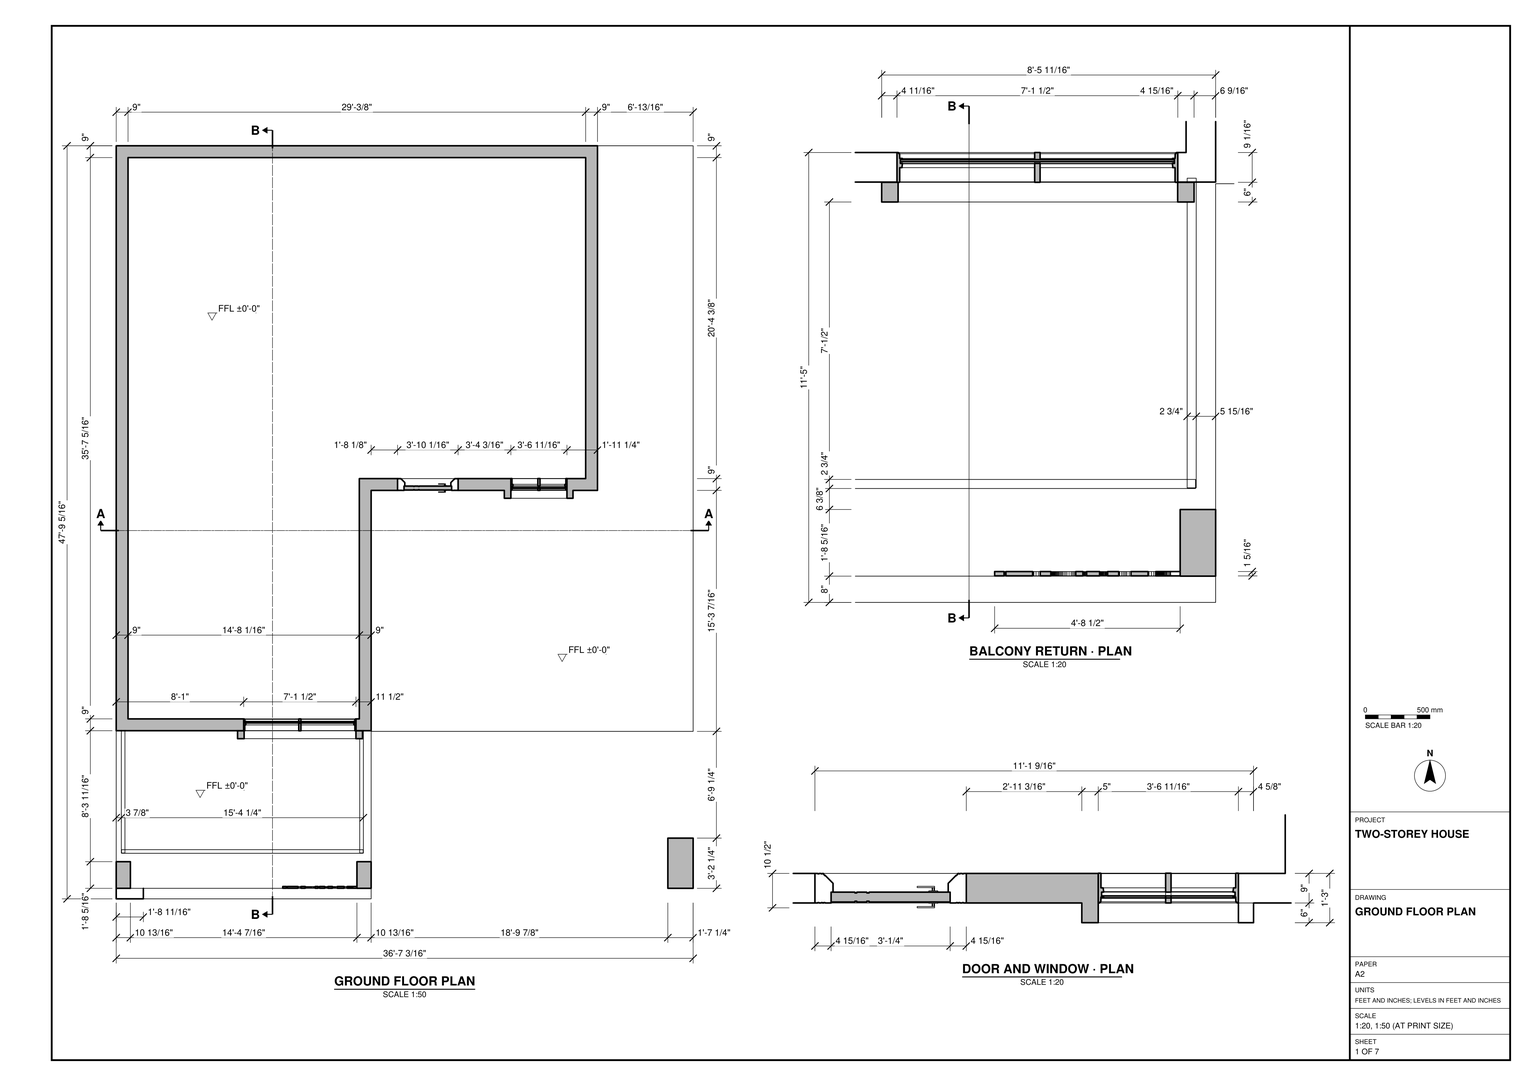
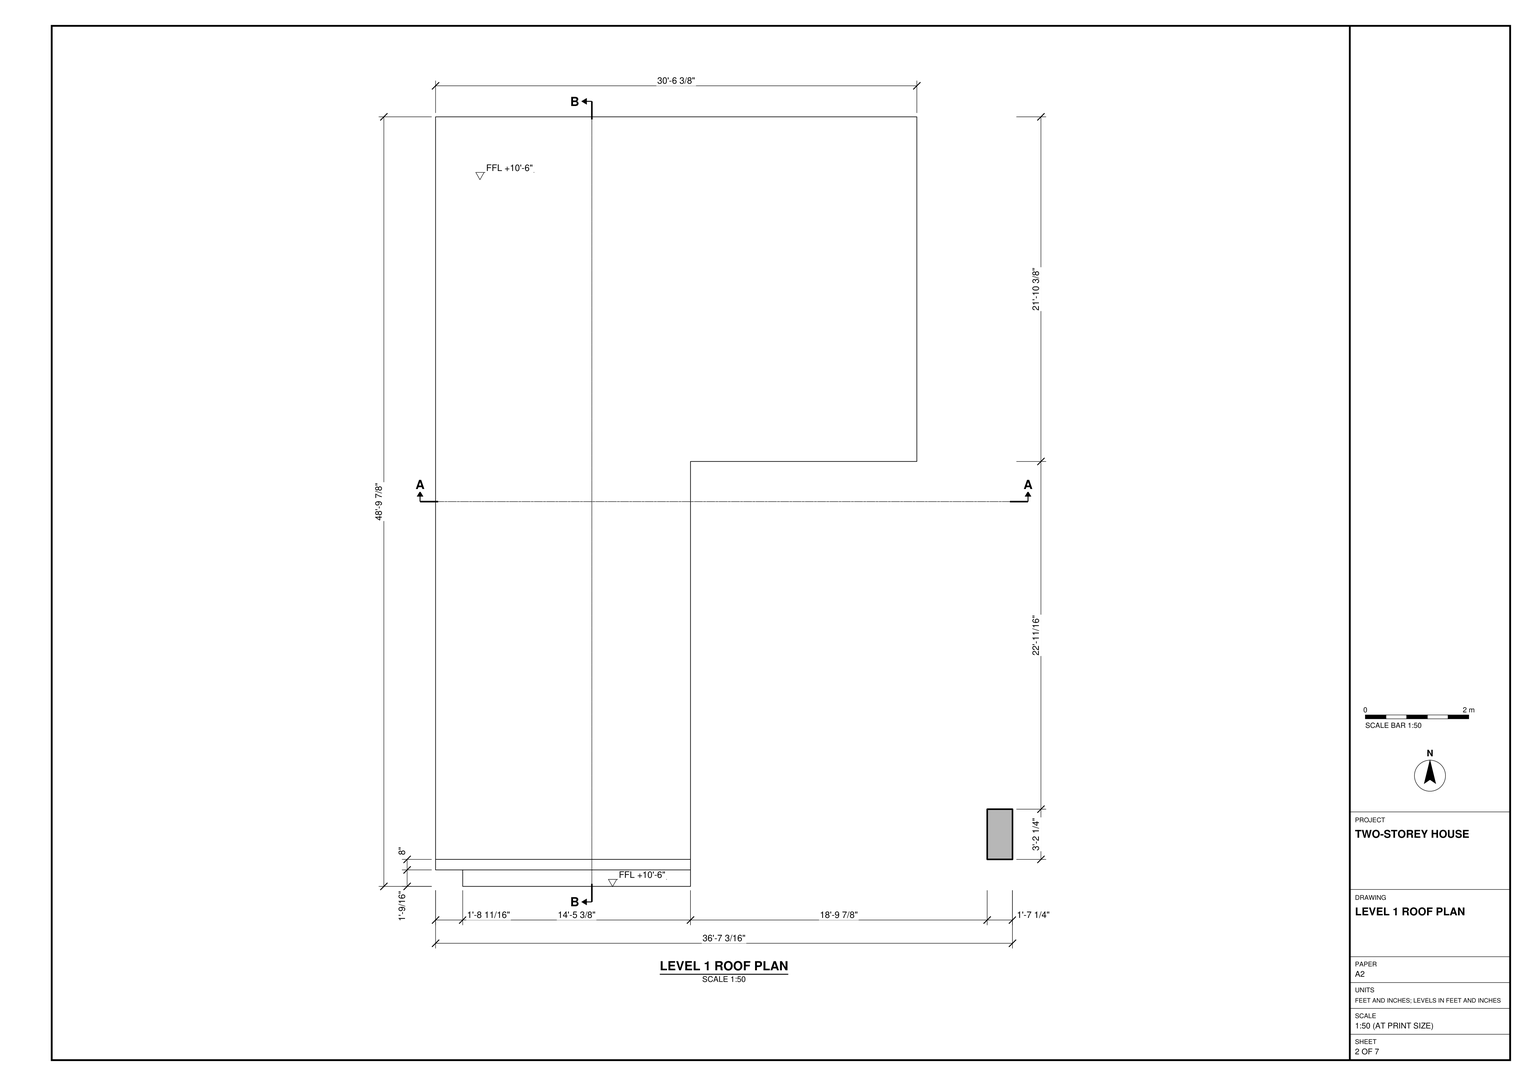
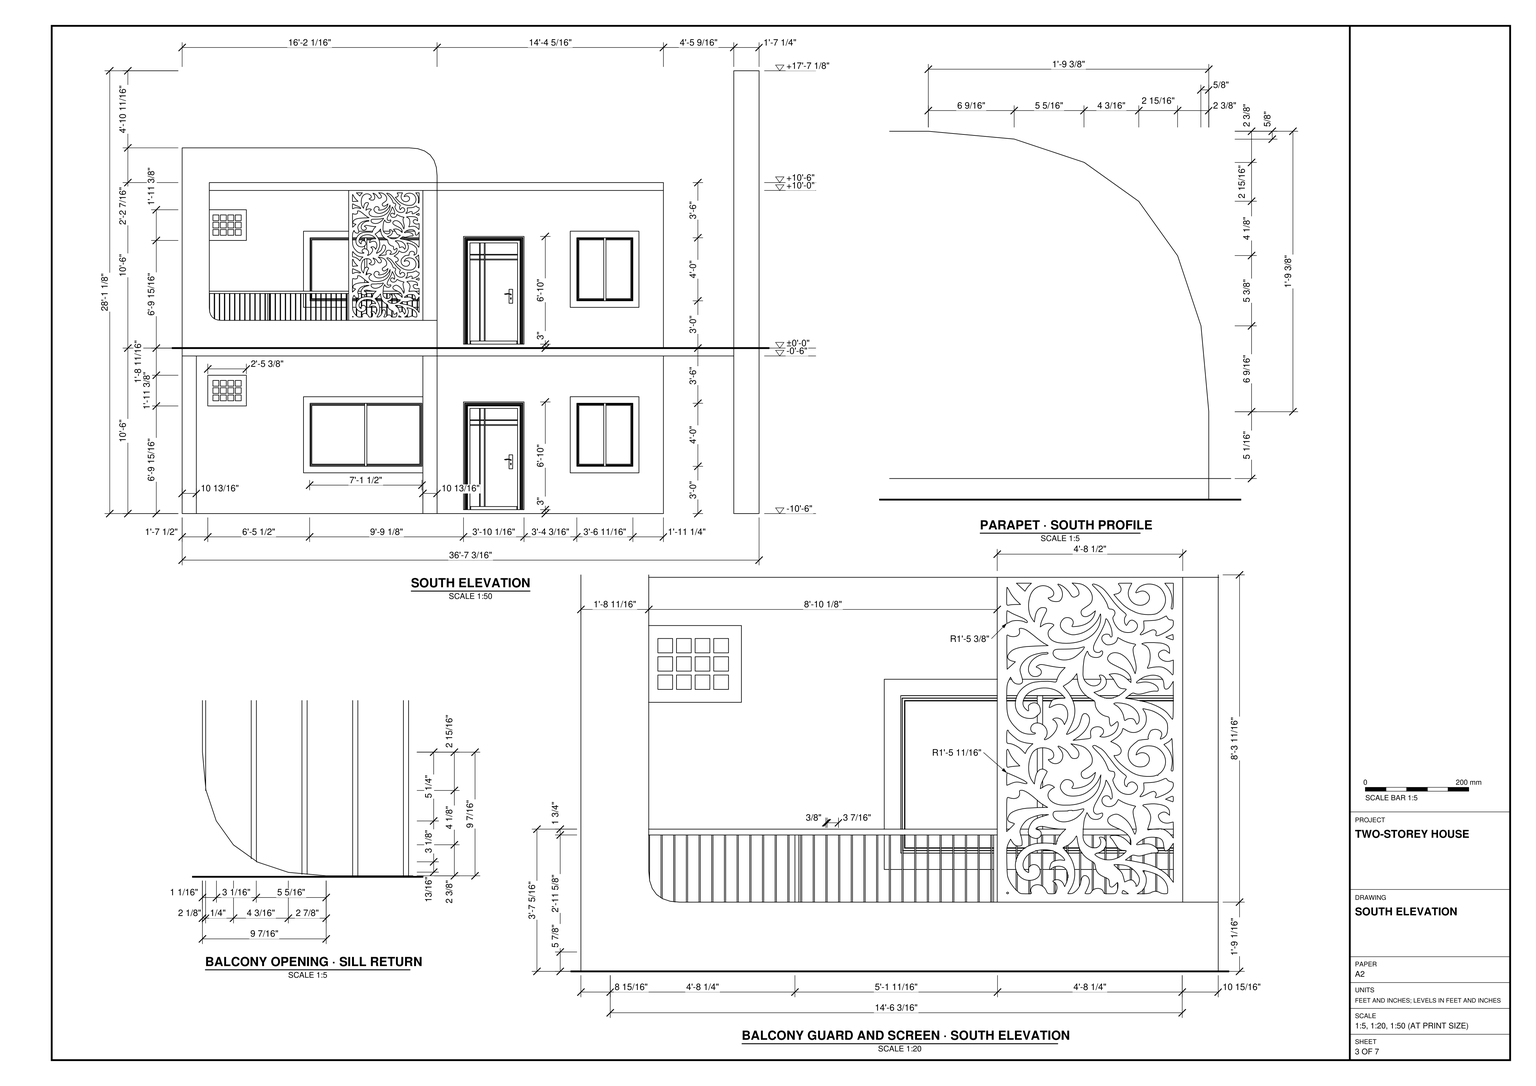
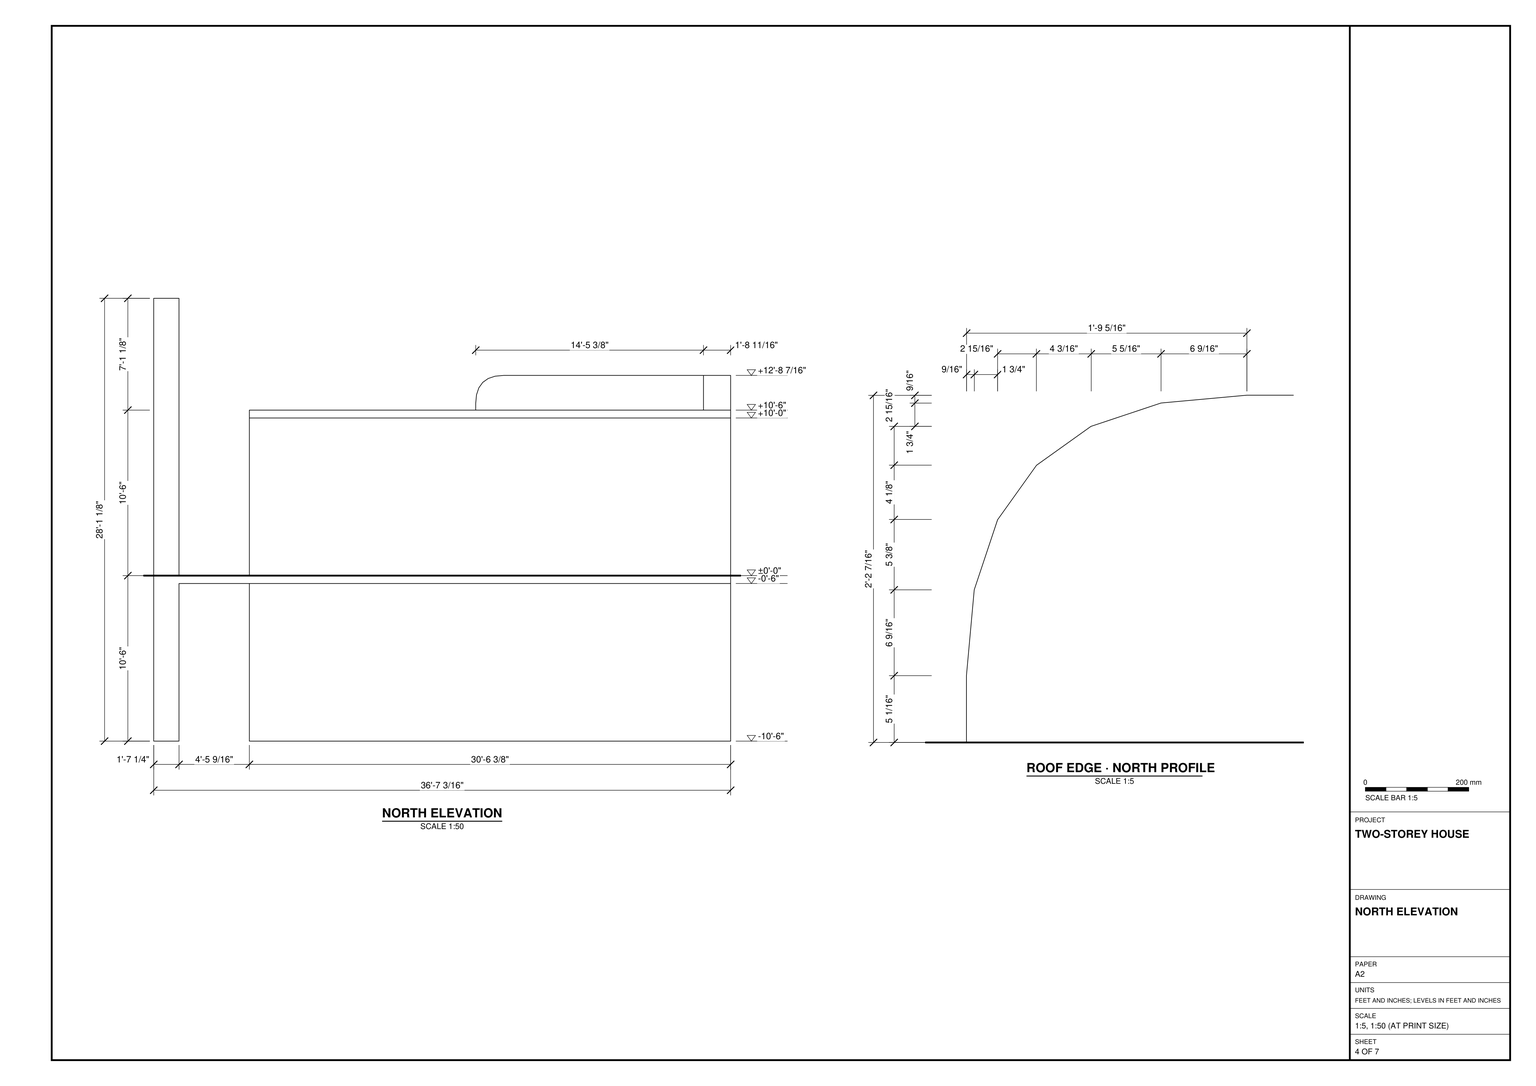
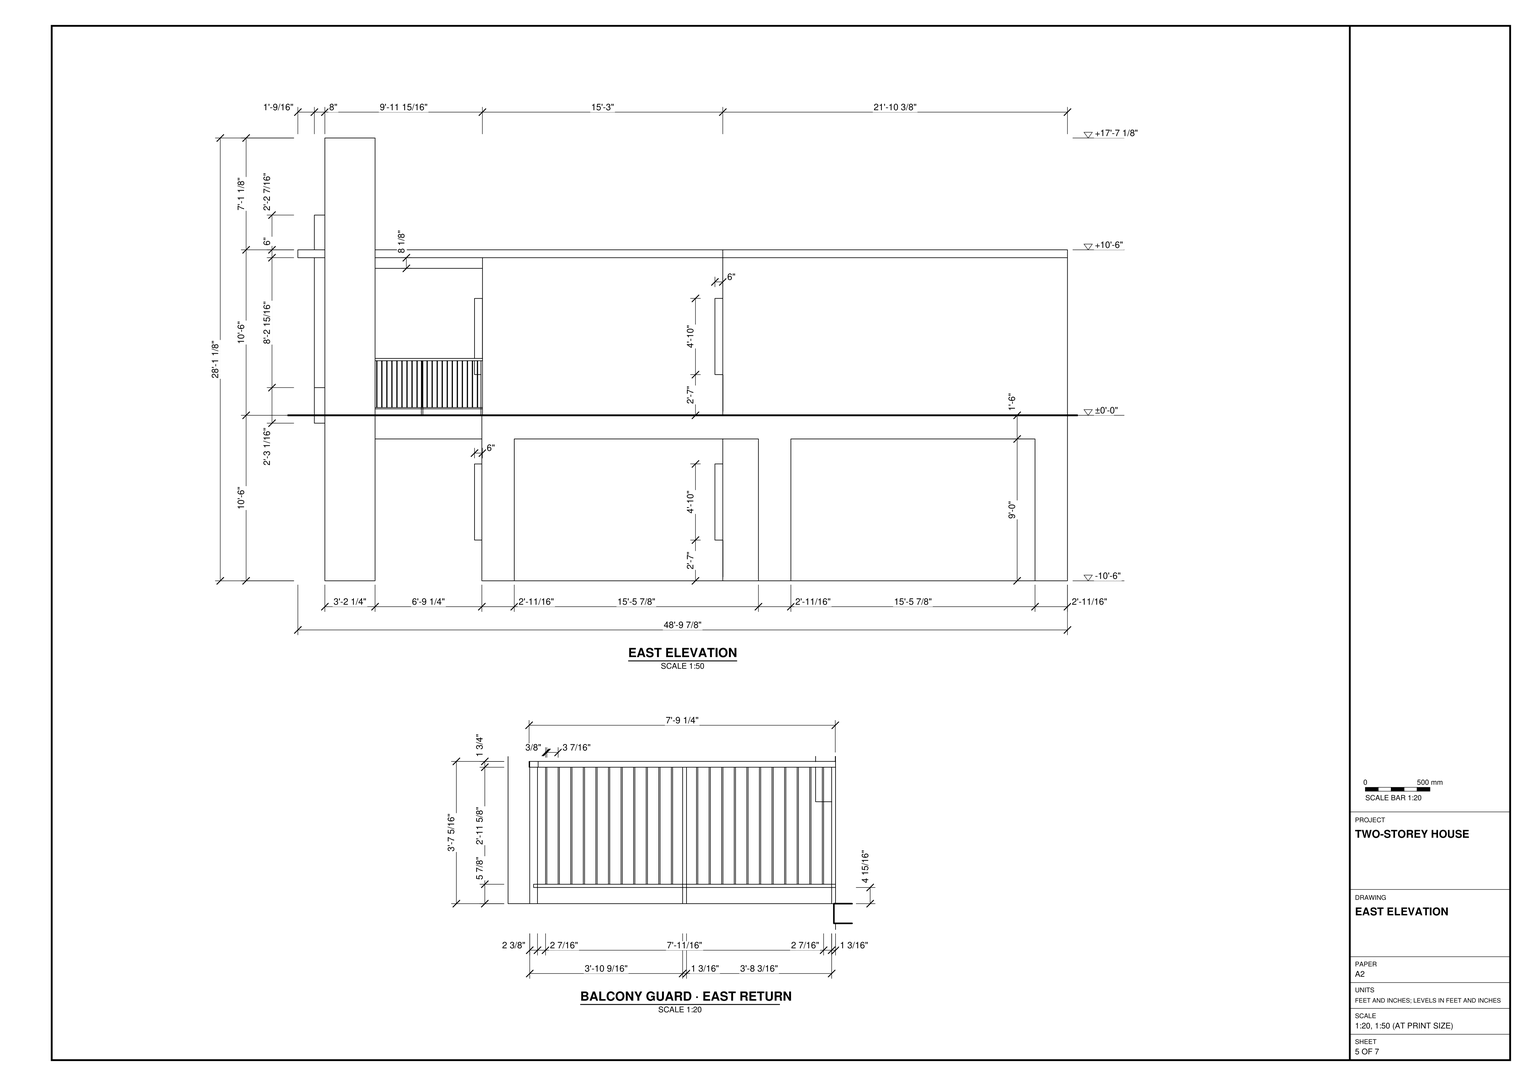
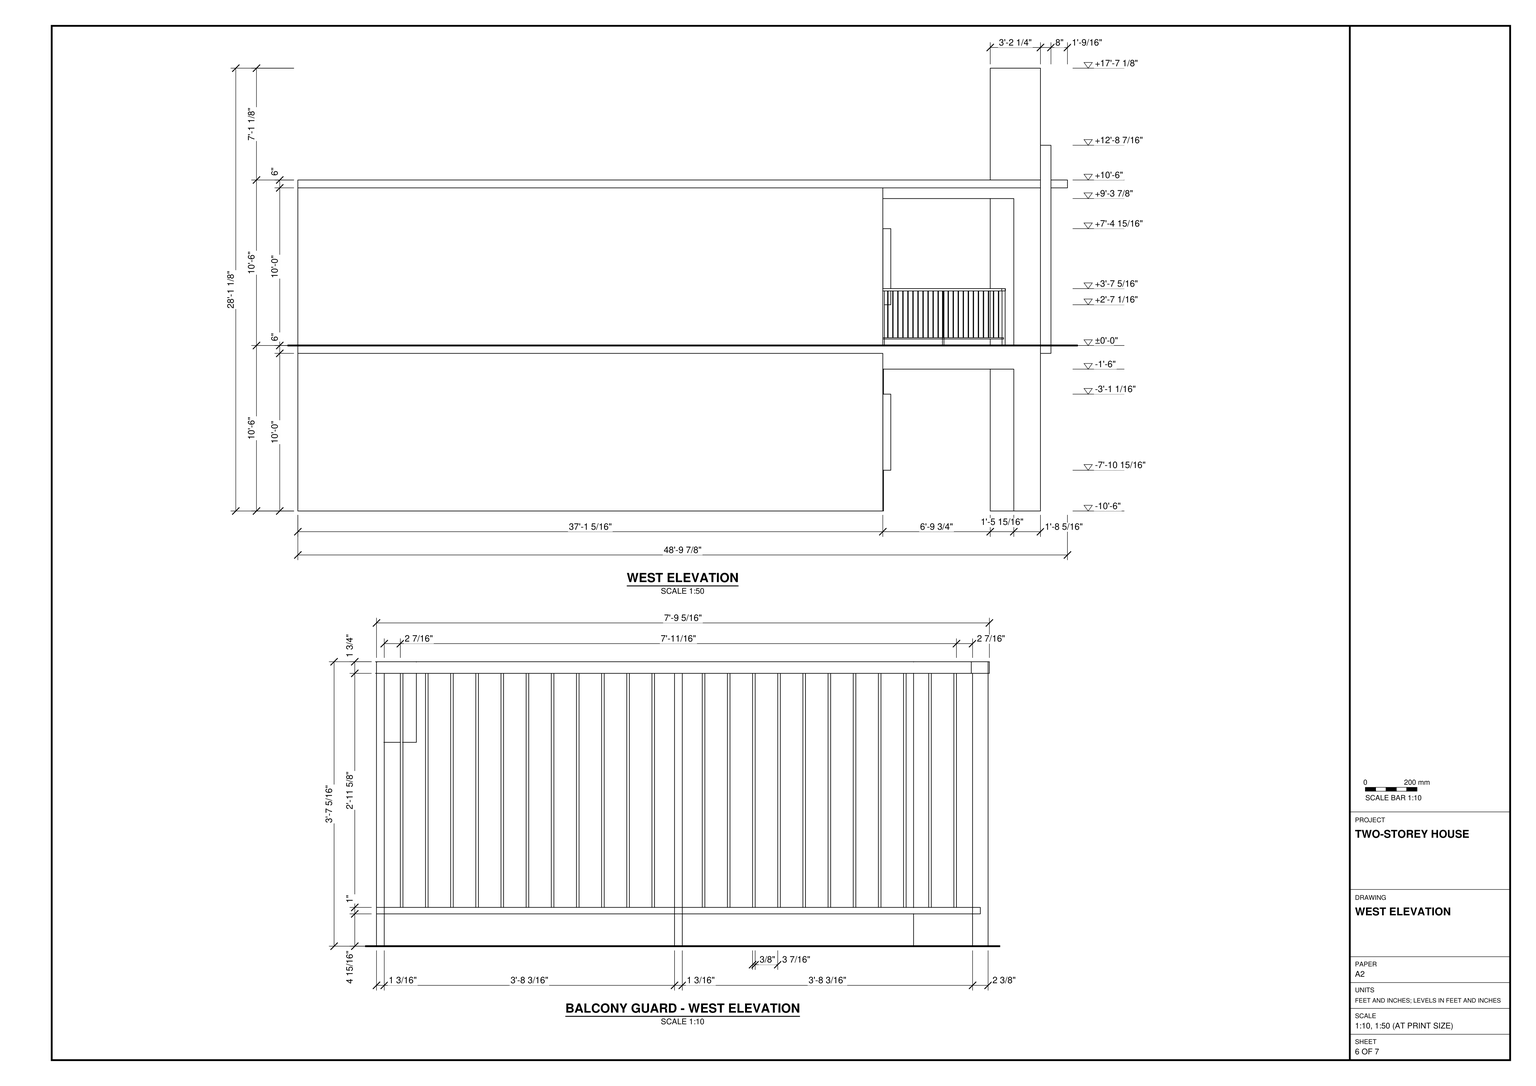
Build the two-storey house in SketchUp from task_files/diagram_01.pdf. Work in feet and inches. The overall width is 36'-7 3/16", the depth is 48'-9 7/8", and the height is 28'-1 1/8". Set the ground-floor finished level to ±0'-0" and the upper-floor finished level to +10'-6".

Lay out the L-shaped shell with the longer wing projecting south on the west side. Use the wall thicknesses shown in plan, including the 9" exterior walls. Follow the stepped outline when forming the floor and flat roof slabs. Include the covered area below the balcony and the separate tall rectangular pier near the southeast corner.

Use the south elevation to position the doors, framed windows and small gridded openings on both storeys. Model the balcony with its solid sill, vertical-bar guard and tall openwork screen at the right end. Follow the enlarged details for the curved sill return and the rounded outer corner of the parapet.

Keep walls, slabs, roof and each furniture or joinery piece shown as separate groups or components, and use components for repeated parts. Any decor or loose items shown may be suitable library components, for example from 3D Warehouse. Save one SketchUp model as output_files/two_storey_house_with_a_screened_front_balcony.skp.

# SketchUp Ruby script. Lengths in inches.
U = 1.inch
M = Sketchup.active_model
def pt(a) = Geom::Point3d.new(a.map { |v| v * U })
def face(e, loops, mat)
  f = e.add_face(loops[0].map { |a| pt(a) })
  loops[1..].each { |l| e.add_face(l.map { |a| pt(a) }).erase! }
  f.material = f.back_material = mat if mat
  f
end
# faces: each face lists its corners as indices into pts; further lists are holes
def faces(e, pts, list, mat = nil) = list.each { |f| face(e, (f[0].is_a?(Array) ? f : [f]).map { |l| l.map { |i| pts[i] } }, mat) }
# xy, xz, yz: faces in a plane at the given z, y or x. An outline is a flat list of corners, or four numbers for a rectangle; further outlines are holes
def ring(l) = l.size == 4 ? [[l[0], l[1]], [l[2], l[1]], [l[2], l[3]], [l[0], l[3]]] : l.each_slice(2).to_a
def flat(e, list, mat, &to3) = list.each { |f| face(e, (f[0].is_a?(Array) ? f : [f]).map { |l| ring(l).map { |u, v| to3.(u, v) } }, mat) }
def xy(e, z, list, mat = nil) = flat(e, list, mat) { |x, y| [x, y, z] }
def xz(e, y, list, mat = nil) = flat(e, list, mat) { |x, z| [x, y, z] }
def yz(e, x, list, mat = nil) = flat(e, list, mat) { |y, z| [x, y, z] }
def lines(e, pts, list) = list.each { |a, b| e.add_line(pt(pts[a]), pt(pts[b])) }
# prism: a flat outline (further loops are holes) pulled along v
def prism(e, loops, v, mat = nil)
  f = face(e, loops, mat); d = Geom::Vector3d.new(v.map { |x| x * U })
  f.pushpull(f.normal.samedirection?(d) ? d.length : -d.length)
end
def box(e, o, s, mat = nil) = prism(e, [[o, [o[0] + s[0], o[1], o[2]], [o[0] + s[0], o[1] + s[1], o[2]], [o[0], o[1] + s[1], o[2]]]], [0, 0, s[2]], mat)
def at(x, y, z, deg = 0) = Geom::Transformation.translation(pt([x, y, z])) * Geom::Transformation.rotation(ORIGIN, Z_AXIS, deg.degrees)
def axes(o, x, y, z) = Geom::Transformation.new([*x, 0, *y, 0, *z, 0, *pt(o).to_a, 1])
def part(name) = M.definitions.add(name)
# library, detail: a bought-in or finely detailed component or shape, given as its bounding box
def library(name, o, s) = part(name).tap { |d| box(d.entities, o, s) }
def detail(e, o, s) = box(e.add_group.entities, o, s)
def put(e, d, t, mat = nil) = e.add_instance(d, t).tap { |i| i.material = mat if mat }
def group(e, t, mat = nil) = e.add_group.tap { |g| g.transformation = t; g.material = mat if mat }.entities
root = M.entities
M.materials.add("[Color B02]").color = [255, 178, 153]
M.materials.add("[Color M08]").color = [30, 30, 30]
M.materials.add("[Metal Silver]").color = [234, 233, 238]
M.materials.add("[Stone Brushed Khaki]").color = [226, 197, 133]
M.materials.add("[Translucent Glass Blue]").color = [100, 149, 237]
M.materials["[Translucent Glass Blue]"].alpha = 0.5
M.materials.add("[Wood Cherry Original]").color = [152, 86, 42]
M.materials.add("[Wood Veneer 01]").color = [120, 70, 37]
c1 = library("CNC jali design",[0,0,0],[196.99,3,392])
c2 = part("Group7\#1")
xy(c2.entities,0,[[-10.75,-7.75,-6.27,-3.375],[-5.08,-7.75,-0.59,-3.375],[0.59,-7.75,5.08,-3.375],[6.27,-7.75,10.75,-3.375],[-10.75,-2.1875,-6.27,2.1875],
  [-5.08,-2.1875,-0.59,2.1875],[0.59,-2.1875,5.08,2.1875],[6.27,-2.1875,10.75,2.1875],[-10.75,3.375,-6.27,7.75],[-5.08,3.375,-0.59,7.75],
  [0.59,3.375,5.08,7.75],[6.27,3.375,10.75,7.75]],"[Translucent Glass Blue]")
c3 = part("Group6\#1")
xy(c3.entities,0,[[[-14.6875,-11.6875,14.6875,11.6875],[6.27,-7.75,10.75,-3.375],[-10.75,-7.75,-6.27,-3.375],[-5.08,-7.75,-0.59,-3.375],[0.59,-7.75,5.08,-3.375],[6.27,-2.1875,10.75,2.1875],[6.27,3.375,10.75,7.75],[-10.75,3.375,-6.27,7.75],[-5.08,3.375,-0.59,7.75],[0.59,-2.1875,5.08,2.1875],[0.59,3.375,5.08,7.75],[-10.75,-2.1875,-6.27,2.1875],[-5.08,-2.1875,-0.59,2.1875]]])
xy(c3.entities,5.875,[[[-14.6875,-11.6875,14.6875,11.6875],[6.27,-7.75,10.75,-3.375],[-10.75,-7.75,-6.27,-3.375],[-5.08,-7.75,-0.59,-3.375],[0.59,-7.75,5.08,-3.375],[6.27,-2.1875,10.75,2.1875],[6.27,3.375,10.75,7.75],[-10.75,3.375,-6.27,7.75],[-5.08,3.375,-0.59,7.75],[0.59,-2.1875,5.08,2.1875],[0.59,3.375,5.08,7.75],[-10.75,-2.1875,-6.27,2.1875],[-5.08,-2.1875,-0.59,2.1875]]],"[Wood Veneer 01]")
xz(c3.entities,-11.6875,[[-14.6875,0,14.6875,5.875]])
xz(c3.entities,-7.75,[[-10.75,0,-6.27,5.875],[-5.08,0,-0.59,5.875],[0.59,0,5.08,5.875],[6.27,0,10.75,5.875]])
xz(c3.entities,-3.375,[[-10.75,0,-6.27,5.875],[-5.08,0,-0.59,5.875],[0.59,0,5.08,5.875],[6.27,0,10.75,5.875]])
xz(c3.entities,-2.1875,[[-10.75,0,-6.27,5.875],[-5.08,0,-0.59,5.875],[0.59,0,5.08,5.875],[6.27,0,10.75,5.875]])
xz(c3.entities,2.1875,[[-10.75,0,-6.27,5.875],[-5.08,0,-0.59,5.875],[0.59,0,5.08,5.875],[6.27,0,10.75,5.875]])
xz(c3.entities,3.375,[[-10.75,0,-6.27,5.875],[-5.08,0,-0.59,5.875],[0.59,0,5.08,5.875],[6.27,0,10.75,5.875]])
xz(c3.entities,7.75,[[-10.75,0,-6.27,5.875],[-5.08,0,-0.59,5.875],[0.59,0,5.08,5.875],[6.27,0,10.75,5.875]])
xz(c3.entities,11.6875,[[-14.6875,0,14.6875,5.875]])
yz(c3.entities,-14.6875,[[-11.6875,0,11.6875,5.875]])
yz(c3.entities,-10.75,[[-7.75,0,-3.375,5.875],[-2.1875,0,2.1875,5.875],[3.375,0,7.75,5.875]])
yz(c3.entities,-6.27,[[-7.75,0,-3.375,5.875],[-2.1875,0,2.1875,5.875],[3.375,0,7.75,5.875]])
yz(c3.entities,-5.08,[[-7.75,0,-3.375,5.875],[-2.1875,0,2.1875,5.875],[3.375,0,7.75,5.875]])
yz(c3.entities,-0.59,[[-7.75,0,-3.375,5.875],[-2.1875,0,2.1875,5.875],[3.375,0,7.75,5.875]])
yz(c3.entities,0.59,[[-7.75,0,-3.375,5.875],[-2.1875,0,2.1875,5.875],[3.375,0,7.75,5.875]])
yz(c3.entities,5.08,[[-7.75,0,-3.375,5.875],[-2.1875,0,2.1875,5.875],[3.375,0,7.75,5.875]])
yz(c3.entities,6.27,[[-7.75,0,-3.375,5.875],[-2.1875,0,2.1875,5.875],[3.375,0,7.75,5.875]])
yz(c3.entities,10.75,[[-7.75,0,-3.375,5.875],[-2.1875,0,2.1875,5.875],[3.375,0,7.75,5.875]])
yz(c3.entities,14.6875,[[-11.6875,0,11.6875,5.875]])
put(c3.entities,c2,at(0,0,2.9375))
c4 = part("Difference\#2")
prism(c4.entities,[[[187.49,6,31.04],[92.37,6,31.04],[92.37,6,88.96],[187.49,6,88.96]],[[182.49,6,36.04],[182.49,6,83.96],[97.37,6,83.96],[97.37,6,36.04]]],[0,-6,0],"[Stone Brushed Khaki]")
xy(c4.entities,0,[[[0,6.07,0,451.38,366.375,451.38,366.375,189.01,194.0625,189.01,194.0625,6.07],[9,15.07,185.0625,15.07,185.0625,198.01,357.375,198.01,357.375,442.38,9,442.38]]])
xy(c4.entities,3,[[214.17,189.01,260.26,198.01]])
xy(c4.entities,31,[[295.4375,183.01,347.73,189.01]],"[Stone Brushed Khaki]")
xy(c4.entities,36,[[97.03,6.07,182.53,15.07]])
xy(c4.entities,36,[[300.4375,183.01,343.125,198.01]],"[Stone Brushed Khaki]")
xy(c4.entities,81.9375,[[19.5,6.07,48.875,15.07]])
xy(c4.entities,84,[[97.03,6.07,182.53,15.07]])
xy(c4.entities,84,[[300.4375,183.01,343.125,198.01]],"[Stone Brushed Khaki]")
xy(c4.entities,85,[[214.17,189.01,260.26,198.01]])
xy(c4.entities,89,[[295.4375,183.01,347.73,189.01]],"[Stone Brushed Khaki]")
xy(c4.entities,105.3125,[[19.5,6.07,48.875,15.07]])
xy(c4.entities,120,[[[0,6.07,194.0625,6.07,194.0625,189.01,366.375,189.01,366.375,451.38,0,451.38],[9,15.07,9,442.38,357.375,442.38,357.375,198.01,185.0625,198.01,185.0625,15.07]]])
xz(c4.entities,6.07,[[[0,0,194.0625,120],[97.03,36,182.53,84],[19.5,81.9375,48.875,105.3125]]])
xz(c4.entities,15.07,[[[9,0,185.0625,120],[97.03,36,182.53,84],[19.5,81.9375,48.875,105.3125]]])
xz(c4.entities,183.01,[[[295.4375,31,347.73,89],[300.4375,36,343.125,84]]],"[Stone Brushed Khaki]")
xz(c4.entities,189.01,[[[194.0625,0,366.375,120],[214.17,3,260.26,85],[295.4375,31,347.73,89]]])
xz(c4.entities,198.01,[[[185.0625,0,357.375,120],[214.17,3,260.26,85],[300.4375,36,343.125,84]]])
xz(c4.entities,442.38,[[9,0,357.375,120]])
xz(c4.entities,451.38,[[0,0,366.375,120]])
yz(c4.entities,0,[[6.07,0,451.38,120]])
yz(c4.entities,9,[[15.07,0,442.38,120]])
yz(c4.entities,19.5,[[6.07,81.9375,15.07,105.3125]])
yz(c4.entities,48.875,[[6.07,81.9375,15.07,105.3125]])
yz(c4.entities,97.03,[[6.07,36,15.07,84]])
yz(c4.entities,182.53,[[6.07,36,15.07,84]])
yz(c4.entities,185.0625,[[15.07,0,198.01,120]])
yz(c4.entities,194.0625,[[6.07,0,189.01,120]])
yz(c4.entities,214.17,[[189.01,3,198.01,85]])
yz(c4.entities,260.26,[[189.01,3,198.01,85]])
yz(c4.entities,295.4375,[[183.01,31,189.01,89]],"[Stone Brushed Khaki]")
yz(c4.entities,300.4375,[[183.01,36,198.01,84]],"[Stone Brushed Khaki]")
yz(c4.entities,343.125,[[183.01,36,198.01,84]],"[Stone Brushed Khaki]")
yz(c4.entities,347.73,[[183.01,31,189.01,89]],"[Stone Brushed Khaki]")
yz(c4.entities,357.375,[[198.01,0,442.38,120]])
yz(c4.entities,366.375,[[189.01,0,451.38,120]])
c5 = part("Group20\#2")
box(c5.entities,[1.02,-2.16,1.02],[40.64,0.63,45.96])
c6 = part("Difference\#1")
put(c6.entities,c4,at(0,0,0))
g1 = group(c6.entities,at(300.4375,189.01,36))
put(g1,c5,at(42.6875,0,0,180),"[Translucent Glass Blue]")
g2 = group(g1,at(42.6875,0,0,180),"[Metal Silver]")
xy(g2,0,[[0,-9,20.52,0],[20.52,-9,22.17,0],[22.17,-9,42.6875,0]])
xy(g2,0.83,[[0.83,-8.93,20.52,-4.61],[22.17,-8.93,41.86,-4.61]])
xy(g2,1.02,[[1.02,-3.3125,20.52,-2.16],[20.52,-3.3125,22.17,-2.16],[22.17,-3.3125,41.66,-2.16]])
xy(g2,1.61,[[1.61,-2.16,20.52,-1.8],[22.17,-2.16,41.07,-1.8]])
xy(g2,1.65,[[1.65,-3.46,20.52,-3.3125],[22.17,-3.46,41.03,-3.3125]])
xy(g2,46.35,[[1.65,-3.46,20.52,-3.3125],[22.17,-3.46,41.03,-3.3125]])
xy(g2,46.39,[[1.61,-2.16,20.52,-1.8],[22.17,-2.16,41.07,-1.8]])
xy(g2,46.98,[[1.02,-3.3125,20.52,-2.16],[20.52,-3.3125,22.17,-2.16],[22.17,-3.3125,41.66,-2.16]])
xy(g2,47.17,[[0.83,-8.93,20.52,-4.61],[22.17,-8.93,41.86,-4.61]])
xy(g2,48,[[0,-9,20.52,0],[20.52,-9,22.17,0],[22.17,-9,42.6875,0]])
xz(g2,-9.07,[[0.04,0.04,20.52,0.04,20.52,0.75,0.75,0.75,0.75,47.25,20.52,47.25,20.52,47.96,0.04,47.96],[20.52,0.04,22.17,47.96],[22.17,0.04,42.65,0.04,42.65,47.96,22.17,47.96,22.17,47.25,41.9375,47.25,41.9375,0.75,22.17,0.75]])
xz(g2,-4.61,[[0.83,0.83,20.52,0.83,20.52,1.5,1.5,1.5,1.5,46.5,20.52,46.5,20.52,47.17,0.83,47.17],[22.17,0.83,41.86,0.83,41.86,47.17,22.17,47.17,22.17,46.5,41.19,46.5,41.19,1.5,22.17,1.5]])
xz(g2,-3.3125,[[1.02,1.02,1.02,46.98,20.52,46.98,20.52,46.35,1.65,46.35,1.65,1.65,20.52,1.65,20.52,1.02],[20.52,1.02,22.17,46.98],[22.17,1.02,22.17,1.65,41.03,1.65,41.03,46.35,22.17,46.35,22.17,46.98,41.66,46.98,41.66,1.02]])
xz(g2,-2.16,[[1.02,1.02,20.52,1.02,20.52,1.61,1.61,1.61,1.61,46.39,20.52,46.39,20.52,46.98,1.02,46.98],[20.52,1.02,22.17,46.98],[22.17,1.02,41.66,1.02,41.66,46.98,22.17,46.98,22.17,46.39,41.07,46.39,41.07,1.61,22.17,1.61]])
xz(g2,-1.8,[[0.83,0.83,0.83,47.17,20.52,47.17,20.52,46.39,1.61,46.39,1.61,1.61,20.52,1.61,20.52,0.83],[22.17,0.83,22.17,1.61,41.07,1.61,41.07,46.39,22.17,46.39,22.17,47.17,41.86,47.17,41.86,0.83]])
xz(g2,-0.36,[[0.59,0.59,0.59,47.41,20.52,47.41,20.52,47.21,0.79,47.21,0.79,0.79,20.52,0.79,20.52,0.59],[22.17,0.59,22.17,0.79,41.9,0.79,41.9,47.21,22.17,47.21,22.17,47.41,42.1,47.41,42.1,0.59]])
xz(g2,0,[[0,0,0,48,20.52,48,20.52,47.61,0.39,47.61,0.39,0.39,20.52,0.39,20.52,0],[20.52,0,22.17,48],[22.17,0,22.17,0.39,42.29,0.39,42.29,47.61,22.17,47.61,22.17,48,42.6875,48,42.6875,0]])
yz(g2,0,[[-9,0,0,48]])
yz(g2,0.83,[[-8.93,0.83,-4.61,47.17]])
yz(g2,1.02,[[-3.3125,1.02,-2.16,46.98]])
yz(g2,1.61,[[-2.16,1.61,-1.8,46.39]])
yz(g2,1.65,[[-3.46,1.65,-3.3125,46.35]])
yz(g2,20.52,[[-9,0,0,0,0,0.39,-0.36,0.59,-0.36,0.79,-1.8,0.83,-1.8,1.61,-2.16,1.61,-2.16,1.02,-3.3125,1.02,-3.3125,1.65,-3.46,1.65,-4.61,1.5,-4.61,0.83,-8.93,0.83,-9.07,0.75,-9.07,0.04],[[-9,0,-9.07,0.04,-9.07,47.96,-9,48,0,48,0,0],[-3.3125,1.02,-2.16,46.98]],[-3.46,46.35,-3.3125,46.35,-3.3125,46.98,-2.16,46.98,-2.16,46.39,-1.8,46.39,-1.8,47.17,-0.36,47.21,-0.36,47.41,0,47.61,0,48,-9,48,-9.07,47.96,-9.07,47.25,-8.93,47.17,-4.61,47.17,-4.61,46.5]])
yz(g2,22.17,[[-9,0,-9.07,0.04,-9.07,0.75,-8.93,0.83,-4.61,0.83,-4.61,1.5,-3.46,1.65,-3.3125,1.65,-3.3125,1.02,-2.16,1.02,-2.16,1.61,-1.8,1.61,-1.8,0.83,-0.36,0.79,-0.36,0.59,0,0.39,0,0],[[-9,0,0,0,0,48,-9,48,-9.07,47.96,-9.07,0.04],[-3.3125,1.02,-2.16,46.98]],[-3.46,46.35,-4.61,46.5,-4.61,47.17,-8.93,47.17,-9.07,47.25,-9.07,47.96,-9,48,0,48,0,47.61,-0.36,47.41,-0.36,47.21,-1.8,47.17,-1.8,46.39,-2.16,46.39,-2.16,46.98,-3.3125,46.98,-3.3125,46.35]])
yz(g2,41.03,[[-3.46,1.65,-3.3125,46.35]])
yz(g2,41.07,[[-2.16,1.61,-1.8,46.39]])
yz(g2,41.66,[[-3.3125,1.02,-2.16,46.98]])
yz(g2,41.86,[[-8.93,0.83,-4.61,47.17]])
yz(g2,42.6875,[[-9,0,0,48]])
p = [[20.52,-9,0],[20.52,-9.07,0.04],[0.04,-9.07,0.04],[0,-9,0],[0.04,-9.07,47.96],[0,-9,48],
  [22.17,-9,0],[22.17,-9.07,0.04],[42.6875,-9,0],[42.65,-9.07,0.04],[42.6875,-9,48],[42.65,-9.07,47.96],
  [20.52,-0.36,0.59],[20.52,0,0.39],[0.39,0,0.39],[0.59,-0.36,0.59],[0.39,0,47.61],[0.59,-0.36,47.41],
  [22.17,0,0.39],[22.17,-0.36,0.59],[42.1,-0.36,0.59],[42.29,0,0.39],[42.1,-0.36,47.41],[42.29,0,47.61],
  [20.52,-9.07,0.75],[20.52,-8.93,0.83],[0.83,-8.93,0.83],[0.75,-9.07,0.75],[0.83,-8.93,47.17],[0.75,-9.07,47.25],
  [22.17,-8.93,0.83],[22.17,-9.07,0.75],[41.9375,-9.07,0.75],[41.86,-8.93,0.83],[41.9375,-9.07,47.25],[41.86,-8.93,47.17],
  [20.52,-1.8,0.83],[20.52,-0.36,0.79],[0.79,-0.36,0.79],[0.83,-1.8,0.83],[0.79,-0.36,47.21],[0.83,-1.8,47.17],
  [22.17,-0.36,0.79],[22.17,-1.8,0.83],[41.86,-1.8,0.83],[41.9,-0.36,0.79],[41.86,-1.8,47.17],[41.9,-0.36,47.21],
  [20.52,-4.61,1.5],[20.52,-3.46,1.65],[1.65,-3.46,1.65],[1.5,-4.61,1.5],[1.65,-3.46,46.35],[1.5,-4.61,46.5],
  [22.17,-3.46,1.65],[22.17,-4.61,1.5],[41.19,-4.61,1.5],[41.03,-3.46,1.65],[41.19,-4.61,46.5],[41.03,-3.46,46.35],
  [20.52,-3.46,46.35],[20.52,-4.61,46.5],[22.17,-4.61,46.5],[22.17,-3.46,46.35],[20.52,-8.93,47.17],[20.52,-9.07,47.25],
  [22.17,-9.07,47.25],[22.17,-8.93,47.17],[20.52,-0.36,47.21],[20.52,-1.8,47.17],[22.17,-1.8,47.17],[22.17,-0.36,47.21],
  [20.52,0,47.61],[20.52,-0.36,47.41],[22.17,-0.36,47.41],[22.17,0,47.61],[20.52,-9.07,47.96],[20.52,-9,48],
  [22.17,-9.07,47.96],[22.17,-9,48]]
faces(g2,p,[[0,1,2,3],[3,2,4,5],[6,7,1,0],[7,6,8,9],[9,8,10,11],[12,13,14,15],[15,14,16,17],[18,19,20,21],
  [21,20,22,23],[24,25,26,27],[27,26,28,29],[30,31,32,33],[33,32,34,35],[36,37,38,39],[39,38,40,41],[42,43,44,45],
  [45,44,46,47],[48,49,50,51],[51,50,52,53],[54,55,56,57],[57,56,58,59],[53,52,60,61],[59,58,62,63],[29,28,64,65],
  [35,34,66,67],[41,40,68,69],[47,46,70,71],[17,16,72,73],[23,22,74,75],[5,4,76,77],[78,79,77,76],[11,10,79,78]])
c7 = library("Group\#3",[0,0,0],[46.09,10.47,82])
c8 = part("Difference")
put(c8.entities,c3,axes([34.1875,5.875,93.625],[1,0,0],[0,0,1],[0,-1,0]),"[Wood Cherry Original]")
put(c8.entities,c6,at(0,-6.07,0))
put(c8.entities,c7,at(214.17,181.47,3))
c9 = part("Group5\#2")
box(c9.entities,[1.02,2.16,1.02],[83.46,0.63,45.96])
c10 = part("Group1\#1")
put(c10.entities,c8,at(97.5625,249.6875,0),"[Color B02]")
g3 = group(c10.entities,at(280.1,258.6875,36,180))
g4 = group(g3,at(0,0,0))
xy(g4,0,[[0,0,41.92,9],[41.92,0,43.58,9],[43.58,0,85.5,9]])
xy(g4,0.83,[[0.83,4.61,41.92,8.93],[43.58,4.61,84.68,8.93]])
xy(g4,1.02,[[1.02,2.16,41.92,3.3125],[41.92,2.16,43.58,3.3125],[43.58,2.16,84.48,3.3125]])
xy(g4,1.61,[[1.61,1.8,41.92,2.16],[43.58,1.8,83.89,2.16]])
xy(g4,1.65,[[1.65,3.3125,41.92,3.46],[43.58,3.3125,83.85,3.46]])
xy(g4,46.35,[[1.65,3.3125,41.92,3.46],[43.58,3.3125,83.85,3.46]])
xy(g4,46.39,[[1.61,1.8,41.92,2.16],[43.58,1.8,83.89,2.16]])
xy(g4,46.98,[[1.02,2.16,41.92,3.3125],[41.92,2.16,43.58,3.3125],[43.58,2.16,84.48,3.3125]])
xy(g4,47.17,[[0.83,4.61,41.92,8.93],[43.58,4.61,84.68,8.93]])
xy(g4,48,[[0,0,41.92,9],[41.92,0,43.58,9],[43.58,0,85.5,9]])
xz(g4,0,[[0,0,41.92,0,41.92,0.39,0.39,0.39,0.39,47.61,41.92,47.61,41.92,48,0,48],[41.92,0,43.58,48],[43.58,0,85.5,0,85.5,48,43.58,48,43.58,47.61,85.11,47.61,85.11,0.39,43.58,0.39]])
xz(g4,0.36,[[0.59,0.59,41.92,0.59,41.92,0.79,0.79,0.79,0.79,47.21,41.92,47.21,41.92,47.41,0.59,47.41],[43.58,0.59,84.91,0.59,84.91,47.41,43.58,47.41,43.58,47.21,84.72,47.21,84.72,0.79,43.58,0.79]])
xz(g4,1.8,[[0.83,0.83,41.92,0.83,41.92,1.61,1.61,1.61,1.61,46.39,41.92,46.39,41.92,47.17,0.83,47.17],[43.58,0.83,84.68,0.83,84.68,47.17,43.58,47.17,43.58,46.39,83.89,46.39,83.89,1.61,43.58,1.61]])
xz(g4,2.16,[[1.02,1.02,1.02,46.98,41.92,46.98,41.92,46.39,1.61,46.39,1.61,1.61,41.92,1.61,41.92,1.02],[41.92,1.02,43.58,46.98],[43.58,1.02,43.58,1.61,83.89,1.61,83.89,46.39,43.58,46.39,43.58,46.98,84.48,46.98,84.48,1.02]])
xz(g4,3.3125,[[1.02,1.02,41.92,1.02,41.92,1.65,1.65,1.65,1.65,46.35,41.92,46.35,41.92,46.98,1.02,46.98],[41.92,1.02,43.58,46.98],[43.58,1.02,84.48,1.02,84.48,46.98,43.58,46.98,43.58,46.35,83.85,46.35,83.85,1.65,43.58,1.65]])
xz(g4,4.61,[[0.83,0.83,0.83,47.17,41.92,47.17,41.92,46.5,1.5,46.5,1.5,1.5,41.92,1.5,41.92,0.83],[43.58,0.83,43.58,1.5,84.01,1.5,84.01,46.5,43.58,46.5,43.58,47.17,84.68,47.17,84.68,0.83]])
xz(g4,9.07,[[0.04,0.04,0.04,47.96,41.92,47.96,41.92,47.25,0.75,47.25,0.75,0.75,41.92,0.75,41.92,0.04],[41.92,0.04,43.58,47.96],[43.58,0.04,43.58,0.75,84.75,0.75,84.75,47.25,43.58,47.25,43.58,47.96,85.46,47.96,85.46,0.04]])
yz(g4,0,[[0,0,9,48]])
yz(g4,0.83,[[4.61,0.83,8.93,47.17]])
yz(g4,1.02,[[2.16,1.02,3.3125,46.98]])
yz(g4,1.61,[[1.8,1.61,2.16,46.39]])
yz(g4,1.65,[[3.3125,1.65,3.46,46.35]])
yz(g4,41.92,[[0,0,9,0,9.07,0.04,9.07,0.75,8.93,0.83,4.61,0.83,4.61,1.5,3.46,1.65,3.3125,1.65,3.3125,1.02,2.16,1.02,2.16,1.61,1.8,1.61,1.8,0.83,0.36,0.79,0.36,0.59,0,0.39],[[0,0,0,48,9,48,9.07,47.96,9.07,0.04,9,0],[2.16,1.02,3.3125,46.98]],[3.3125,46.35,3.46,46.35,4.61,46.5,4.61,47.17,8.93,47.17,9.07,47.25,9.07,47.96,9,48,0,48,0,47.61,0.36,47.41,0.36,47.21,1.8,47.17,1.8,46.39,2.16,46.39,2.16,46.98,3.3125,46.98]])
yz(g4,43.58,[[0,0,0,0.39,0.36,0.59,0.36,0.79,1.8,0.83,1.8,1.61,2.16,1.61,2.16,1.02,3.3125,1.02,3.3125,1.65,3.46,1.65,4.61,1.5,4.61,0.83,8.93,0.83,9.07,0.75,9.07,0.04,9,0],[[0,0,9,0,9.07,0.04,9.07,47.96,9,48,0,48],[2.16,1.02,3.3125,46.98]],[3.3125,46.35,3.3125,46.98,2.16,46.98,2.16,46.39,1.8,46.39,1.8,47.17,0.36,47.21,0.36,47.41,0,47.61,0,48,9,48,9.07,47.96,9.07,47.25,8.93,47.17,4.61,47.17,4.61,46.5,3.46,46.35]])
yz(g4,83.85,[[3.3125,1.65,3.46,46.35]])
yz(g4,83.89,[[1.8,1.61,2.16,46.39]])
yz(g4,84.48,[[2.16,1.02,3.3125,46.98]])
yz(g4,84.68,[[4.61,0.83,8.93,47.17]])
yz(g4,85.5,[[0,0,9,48]])
p = [[41.92,9.07,0.04],[41.92,9,0],[0,9,0],[0.04,9.07,0.04],[0,9,48],[0.04,9.07,47.96],
  [43.58,9.07,0.04],[43.58,9,0],[85.46,9.07,0.04],[85.5,9,0],[85.46,9.07,47.96],[85.5,9,48],
  [41.92,0,0.39],[41.92,0.36,0.59],[0.59,0.36,0.59],[0.39,0,0.39],[0.59,0.36,47.41],[0.39,0,47.61],
  [43.58,0.36,0.59],[43.58,0,0.39],[85.11,0,0.39],[84.91,0.36,0.59],[85.11,0,47.61],[84.91,0.36,47.41],
  [41.92,8.93,0.83],[41.92,9.07,0.75],[0.75,9.07,0.75],[0.83,8.93,0.83],[0.75,9.07,47.25],[0.83,8.93,47.17],
  [43.58,9.07,0.75],[43.58,8.93,0.83],[84.68,8.93,0.83],[84.75,9.07,0.75],[84.68,8.93,47.17],[84.75,9.07,47.25],
  [41.92,0.36,0.79],[41.92,1.8,0.83],[0.83,1.8,0.83],[0.79,0.36,0.79],[0.83,1.8,47.17],[0.79,0.36,47.21],
  [43.58,1.8,0.83],[43.58,0.36,0.79],[84.72,0.36,0.79],[84.68,1.8,0.83],[84.72,0.36,47.21],[84.68,1.8,47.17],
  [41.92,3.46,1.65],[41.92,4.61,1.5],[1.5,4.61,1.5],[1.65,3.46,1.65],[1.5,4.61,46.5],[1.65,3.46,46.35],
  [43.58,4.61,1.5],[43.58,3.46,1.65],[83.85,3.46,1.65],[84.01,4.61,1.5],[83.85,3.46,46.35],[84.01,4.61,46.5],
  [41.92,4.61,46.5],[41.92,3.46,46.35],[43.58,3.46,46.35],[43.58,4.61,46.5],[41.92,1.8,47.17],[41.92,0.36,47.21],
  [43.58,0.36,47.21],[43.58,1.8,47.17],[41.92,9.07,47.25],[41.92,8.93,47.17],[43.58,8.93,47.17],[43.58,9.07,47.25],
  [41.92,0.36,47.41],[41.92,0,47.61],[43.58,0,47.61],[43.58,0.36,47.41],[41.92,9,48],[41.92,9.07,47.96],
  [43.58,9,48],[43.58,9.07,47.96]]
faces(g4,p,[[0,1,2,3],[3,2,4,5],[1,0,6,7],[7,6,8,9],[9,8,10,11],[12,13,14,15],[15,14,16,17],[18,19,20,21],
  [21,20,22,23],[24,25,26,27],[27,26,28,29],[30,31,32,33],[33,32,34,35],[36,37,38,39],[39,38,40,41],[42,43,44,45],
  [45,44,46,47],[48,49,50,51],[51,50,52,53],[54,55,56,57],[57,56,58,59],[53,52,60,61],[59,58,62,63],[41,40,64,65],
  [47,46,66,67],[29,28,68,69],[35,34,70,71],[17,16,72,73],[23,22,74,75],[5,4,76,77],[77,76,78,79],[11,10,79,78]])
put(g3,c9,at(0,0,0),"[Translucent Glass Blue]")
c11 = part("Group26\#1")
box(c11.entities,[101.65,248.51,126],[2.36,2.36,41.54])
c12 = part("Group27\#1")
box(c12.entities,[101.65,156.57,126],[2.36,2.36,41.54])
c13 = part("Group28\#1")
box(c13.entities,[101.65,203.13,126],[2.36,1.18,41.54])
c14 = part("Group29\#1")
box(c14.entities,[101.45,156.57,167.54],[2.76,94.3,1.77])
c15 = part("Group30\#1")
box(c15.entities,[101.84,157.75,130.92],[1.97,91.9375,0.99])
c16 = part("Group31\#1")
box(c16.entities,[102.04,245.66,131.91],[1.58,0.39,35.63])
box(c16.entities,[102.04,241.83,131.91],[1.58,0.39,35.63])
box(c16.entities,[102.04,238,131.91],[1.58,0.39,35.63])
box(c16.entities,[102.04,234.17,131.91],[1.58,0.39,35.63])
box(c16.entities,[102.04,230.34,131.91],[1.58,0.39,35.63])
box(c16.entities,[102.04,226.51,131.91],[1.58,0.39,35.63])
box(c16.entities,[102.04,222.68,131.91],[1.58,0.39,35.63])
box(c16.entities,[102.04,218.84,131.91],[1.58,0.4,35.63])
box(c16.entities,[102.04,215.01,131.91],[1.58,0.4,35.63])
box(c16.entities,[102.04,211.18,131.91],[1.58,0.4,35.63])
box(c16.entities,[102.04,207.35,131.91],[1.58,0.4,35.63])
box(c16.entities,[102.04,203.52,131.91],[1.58,0.4,35.63])
box(c16.entities,[102.04,199.69,131.91],[1.58,0.39,35.63])
box(c16.entities,[102.04,195.86,131.91],[1.58,0.39,35.63])
box(c16.entities,[102.04,192.03,131.91],[1.58,0.39,35.63])
box(c16.entities,[102.04,188.2,131.91],[1.58,0.39,35.63])
box(c16.entities,[102.04,184.37,131.91],[1.58,0.39,35.63])
box(c16.entities,[102.04,180.54,131.91],[1.58,0.39,35.63])
box(c16.entities,[102.04,176.71,131.91],[1.58,0.39,35.63])
box(c16.entities,[102.04,172.875,131.91],[1.58,0.4,35.63])
box(c16.entities,[102.04,169.05,131.91],[1.58,0.39,35.63])
box(c16.entities,[102.04,165.21,131.91],[1.58,0.4,35.63])
box(c16.entities,[102.04,161.38,131.91],[1.58,0.4,35.63])
c17 = part("Group33\#1")
box(c17.entities,[283.15,156.57,126],[2.36,2.36,41.54])
c18 = part("Group33\#2")
box(c18.entities,[283.15,248.51,126],[2.36,2.36,41.54])
c19 = part("Group34\#1")
box(c19.entities,[283.15,203.13,126],[2.36,1.18,41.54])
c20 = part("Group35\#1")
box(c20.entities,[282.95,156.57,167.54],[2.76,94.3,1.77])
c21 = part("Group36\#1")
box(c21.entities,[283.34,157.75,130.92],[1.97,91.9375,0.99])
c22 = part("Group37\#1")
box(c22.entities,[283.54,161.38,131.91],[1.58,0.4,35.63])
box(c22.entities,[283.54,165.21,131.91],[1.58,0.4,35.63])
box(c22.entities,[283.54,169.05,131.91],[1.58,0.39,35.63])
box(c22.entities,[283.54,172.875,131.91],[1.58,0.4,35.63])
box(c22.entities,[283.54,176.71,131.91],[1.58,0.39,35.63])
box(c22.entities,[283.54,180.54,131.91],[1.58,0.39,35.63])
box(c22.entities,[283.54,184.37,131.91],[1.58,0.39,35.63])
box(c22.entities,[283.54,188.2,131.91],[1.58,0.39,35.63])
box(c22.entities,[283.54,192.03,131.91],[1.58,0.39,35.63])
box(c22.entities,[283.54,195.86,131.91],[1.58,0.39,35.63])
box(c22.entities,[283.54,199.69,131.91],[1.58,0.39,35.63])
box(c22.entities,[283.54,203.52,131.91],[1.58,0.4,35.63])
box(c22.entities,[283.54,207.35,131.91],[1.58,0.4,35.63])
box(c22.entities,[283.54,211.18,131.91],[1.58,0.4,35.63])
box(c22.entities,[283.54,215.01,131.91],[1.58,0.4,35.63])
box(c22.entities,[283.54,218.84,131.91],[1.58,0.4,35.63])
box(c22.entities,[283.54,222.68,131.91],[1.58,0.39,35.63])
box(c22.entities,[283.54,226.51,131.91],[1.58,0.39,35.63])
box(c22.entities,[283.54,230.34,131.91],[1.58,0.39,35.63])
box(c22.entities,[283.54,234.17,131.91],[1.58,0.39,35.63])
box(c22.entities,[283.54,238,131.91],[1.58,0.39,35.63])
box(c22.entities,[283.54,241.83,131.91],[1.58,0.39,35.63])
box(c22.entities,[283.54,245.66,131.91],[1.58,0.39,35.63])
c23 = part("Group40\#1")
box(c23.entities,[162.74,156.57,126],[1.18,2.36,41.54])
box(c23.entities,[223.24,156.57,126],[1.18,2.36,41.54])
c24 = part("Group41\#1")
box(c24.entities,[101.65,156.37,167.54],[183.86,2.76,1.77])
c25 = part("Group42\#1")
box(c25.entities,[102.83,156.77,130.92],[181.5,1.96,0.99])
c26 = library("Group43\#1",[106.49,156.96,131.91],[174.17,1.58,35.63])
xy(root,120,[[0,12.5625,20.66,20.5625],[20.66,12.5625,194.0625,20.5625]])
xy(root,147.09,[[30.09,12.5625,194.0625,20.5625]],"[Color M08]")
xy(root,252,[[20.66,12.5625,194.0625,20.5625]])
xy(root,278.4375,[[0,12.5625,172.73,20.5625]],"[Color M08]")
xz(root,12.5625,[[0,120,194.0625,120,194.0625,147.09,30.09,147.09,27.21,147.35,24.85,148.13,23.02,149.44,21.71,151.27,20.92,153.63,20.66,156.51,20.66,252,194.0625,252,194.0625,257.1,193.47,263.625,191.69,268.96,188.73,273.1,184.58,276.07,179.25,277.84,172.73,278.4375,0,278.4375]],"[Color M08]")
xz(root,20.5625,[[20.66,252,20.66,278.4375,172.73,278.4375,179.25,277.84,184.58,276.07,188.73,273.1,191.69,268.96,193.47,263.625,194.0625,257.1,194.0625,252]])
yz(root,0,[[12.5625,120,20.5625,278.4375]],"[Color M08]")
yz(root,20.66,[[12.5625,156.51,20.5625,252]],"[Color M08]")
yz(root,194.0625,[[12.5625,120,20.5625,147.09],[12.5625,252,20.5625,257.1]],"[Color M08]")
p = [[30.09,12.5625,147.09],[30.09,20.5625,147.09],[27.21,20.5625,147.35],[27.21,12.5625,147.35],[24.85,20.5625,148.13],[24.85,12.5625,148.13],
  [23.02,20.5625,149.44],[23.02,12.5625,149.44],[21.71,20.5625,151.27],[21.71,12.5625,151.27],[20.92,20.5625,153.63],[20.92,12.5625,153.63],
  [20.66,20.5625,156.51],[20.66,12.5625,156.51],[194.0625,12.5625,257.1],[194.0625,20.5625,257.1],[193.47,20.5625,263.625],[193.47,12.5625,263.625],
  [191.69,20.5625,268.96],[191.69,12.5625,268.96],[188.73,20.5625,273.1],[188.73,12.5625,273.1],[184.58,20.5625,276.07],[184.58,12.5625,276.07],
  [179.25,20.5625,277.84],[179.25,12.5625,277.84],[172.73,20.5625,278.4375],[172.73,12.5625,278.4375]]
faces(root,p,[[0,1,2,3],[3,2,4,5],[5,4,6,7],[7,6,8,9],[9,8,10,11],[11,10,12,13],[14,15,16,17],[17,16,18,19],
  [19,18,20,21],[21,20,22,23],[23,22,24,25],[25,24,26,27]],"[Color M08]")
put(root,c1,axes([126.77,20.63,147.09],[0.28678,0,0],[0,0.44223,0],[0,0,0.25426]))
put(root,c10,at(-97.5625,-109.125,0))
g5 = group(root,at(0,140.5625,120))
box(g5,[419.94,-120,-120],[19.25,38.23,337.125])
xy(g5,-120,[[0,-120,10.8,-99.71],[183.26,-120,194.0625,-99.71],[419.94,-0.5,439.1875,24.1875],[419.94,210.0625,439.1875,234.75],[419.94,420.625,439.1875,445.3125]])
xy(g5,-12,[[0,-99.71,10.8,0],[183.26,-99.71,194.0625,0],[419.94,24.1875,439.1875,210.0625],[419.94,234.75,439.1875,420.625]])
xy(g5,0,[[10.8,-120,10.8,0,0,0,0,445.3125,419.94,445.3125,419.94,-0.5,194.0625,-0.5,194.0625,0,183.26,0,183.26,-120]])
xy(g5,6,[[10.8,-120,183.26,-120,183.26,-99.71,194.0625,-99.71,194.0625,-0.5,439.1875,-0.5,439.1875,445.3125,0,445.3125,0,-99.71,10.8,-99.71]])
xy(g5,117.87,[[0,-99.71,10.8,0],[183.26,-99.71,194.0625,0]])
xy(g5,126,[[0,-120,10.8,0],[183.26,-120,194.0625,0]])
xz(g5,-120,[[0,-120,10.8,-120,10.8,0,183.26,0,183.26,-120,194.0625,-120,194.0625,126,183.26,126,183.26,6,10.8,6,10.8,126,0,126]])
xz(g5,-99.71,[[0,-120,10.8,-12],[183.26,-120,194.0625,-12],[0,6,10.8,117.87],[183.26,6,194.0625,117.87]])
xz(g5,-0.5,[[419.94,-120,439.1875,-120,439.1875,6,194.0625,6,194.0625,0,419.94,0]])
xz(g5,0,[[0,-12,10.8,0],[183.26,-12,194.0625,0],[0,117.87,10.8,126],[183.26,117.87,194.0625,126]])
xz(g5,24.1875,[[419.94,-120,439.1875,-12]])
xz(g5,210.0625,[[419.94,-120,439.1875,-12]])
xz(g5,234.75,[[419.94,-120,439.1875,-12]])
xz(g5,420.625,[[419.94,-120,439.1875,-12]])
xz(g5,445.3125,[[419.94,-120,419.94,0,0,0,0,6,439.1875,6,439.1875,-120]])
yz(g5,0,[[-120,-120,-120,126,0,126,0,117.87,-99.71,117.87,-99.71,6,445.3125,6,445.3125,0,0,0,0,-12,-99.71,-12,-99.71,-120]])
yz(g5,10.8,[[-120,-120,-99.71,-120,-99.71,-12,0,-12,0,0,-120,0],[-120,6,-99.71,6,-99.71,117.87,0,117.87,0,126,-120,126]])
yz(g5,183.26,[[-120,-120,-120,0,0,0,0,-12,-99.71,-12,-99.71,-120],[-120,6,-120,126,0,126,0,117.87,-99.71,117.87,-99.71,6]])
yz(g5,194.0625,[[-120,-120,-99.71,-120,-99.71,-12,0,-12,0,0,-0.5,0,-0.5,6,-99.71,6,-99.71,117.87,0,117.87,0,126,-120,126]])
yz(g5,419.94,[[-0.5,-120,-0.5,0,445.3125,0,445.3125,-120,420.625,-120,420.625,-12,234.75,-12,234.75,-120,210.0625,-120,210.0625,-12,24.1875,-12,24.1875,-120]])
yz(g5,439.1875,[[-0.5,-120,24.1875,-120,24.1875,-12,210.0625,-12,210.0625,-120,234.75,-120,234.75,-12,420.625,-12,420.625,-120,445.3125,-120,445.3125,6,-0.5,6]])
put(root,c10,at(-97.5625,-109.125,126))
g6 = group(root,at(0,140.5625,246))
prism(g6,[[[0,-120,0],[0,445.3125,0],[366.375,445.3125,0],[366.375,182.9375,0],[194.0625,182.9375,0],[194.0625,-140.5625,0],[20.66,-140.5625,0],[20.66,-120,0]]],[0,0,6])
put(root,c11,at(-97.5625,-109.125,0))
put(root,c12,at(-97.5625,-109.125,0))
put(root,c13,at(-97.5625,-109.125,0))
put(root,c14,at(-97.5625,-109.125,0))
put(root,c15,at(-97.5625,-109.125,0))
put(root,c16,at(-97.5625,-109.125,0))
put(root,c17,at(-97.5625,-109.125,0))
put(root,c18,at(-97.5625,-109.125,0))
put(root,c19,at(-97.5625,-109.125,0))
put(root,c20,at(-97.5625,-109.125,0))
put(root,c21,at(-97.5625,-109.125,0))
put(root,c22,at(-97.5625,-109.125,0))
put(root,c23,at(-97.5625,-109.125,0))
put(root,c24,at(-97.5625,-109.125,0))
put(root,c25,at(-97.5625,-109.125,0))
put(root,c26,at(-97.5625,-109.125,0))
